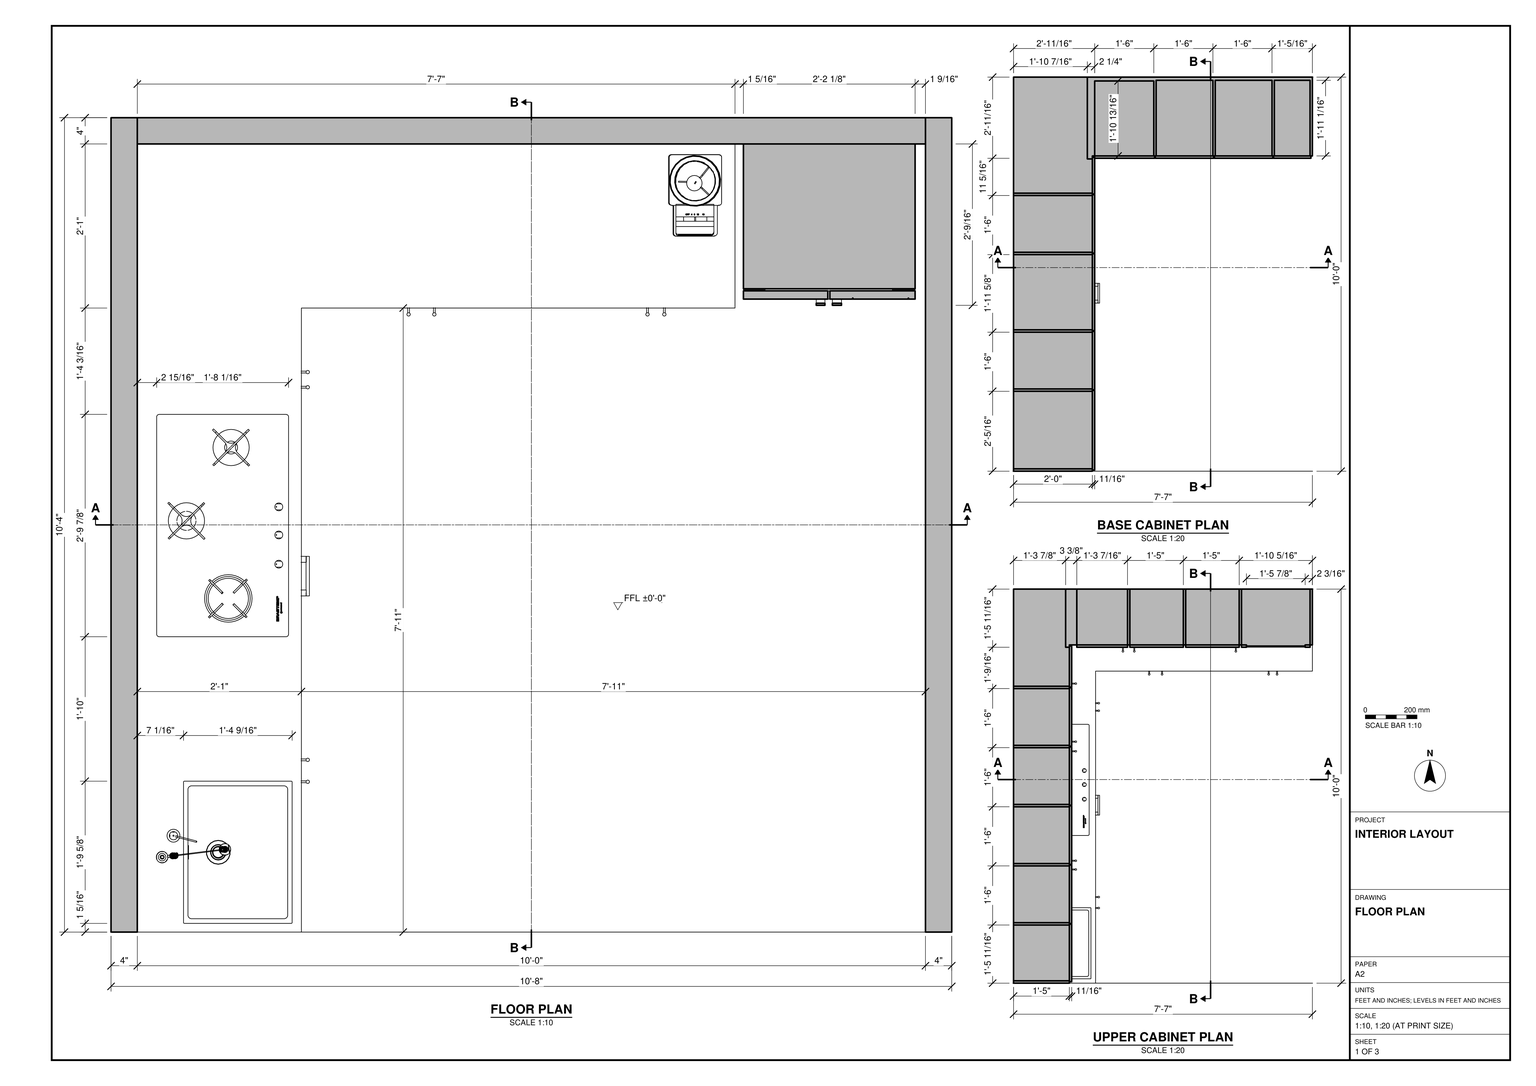
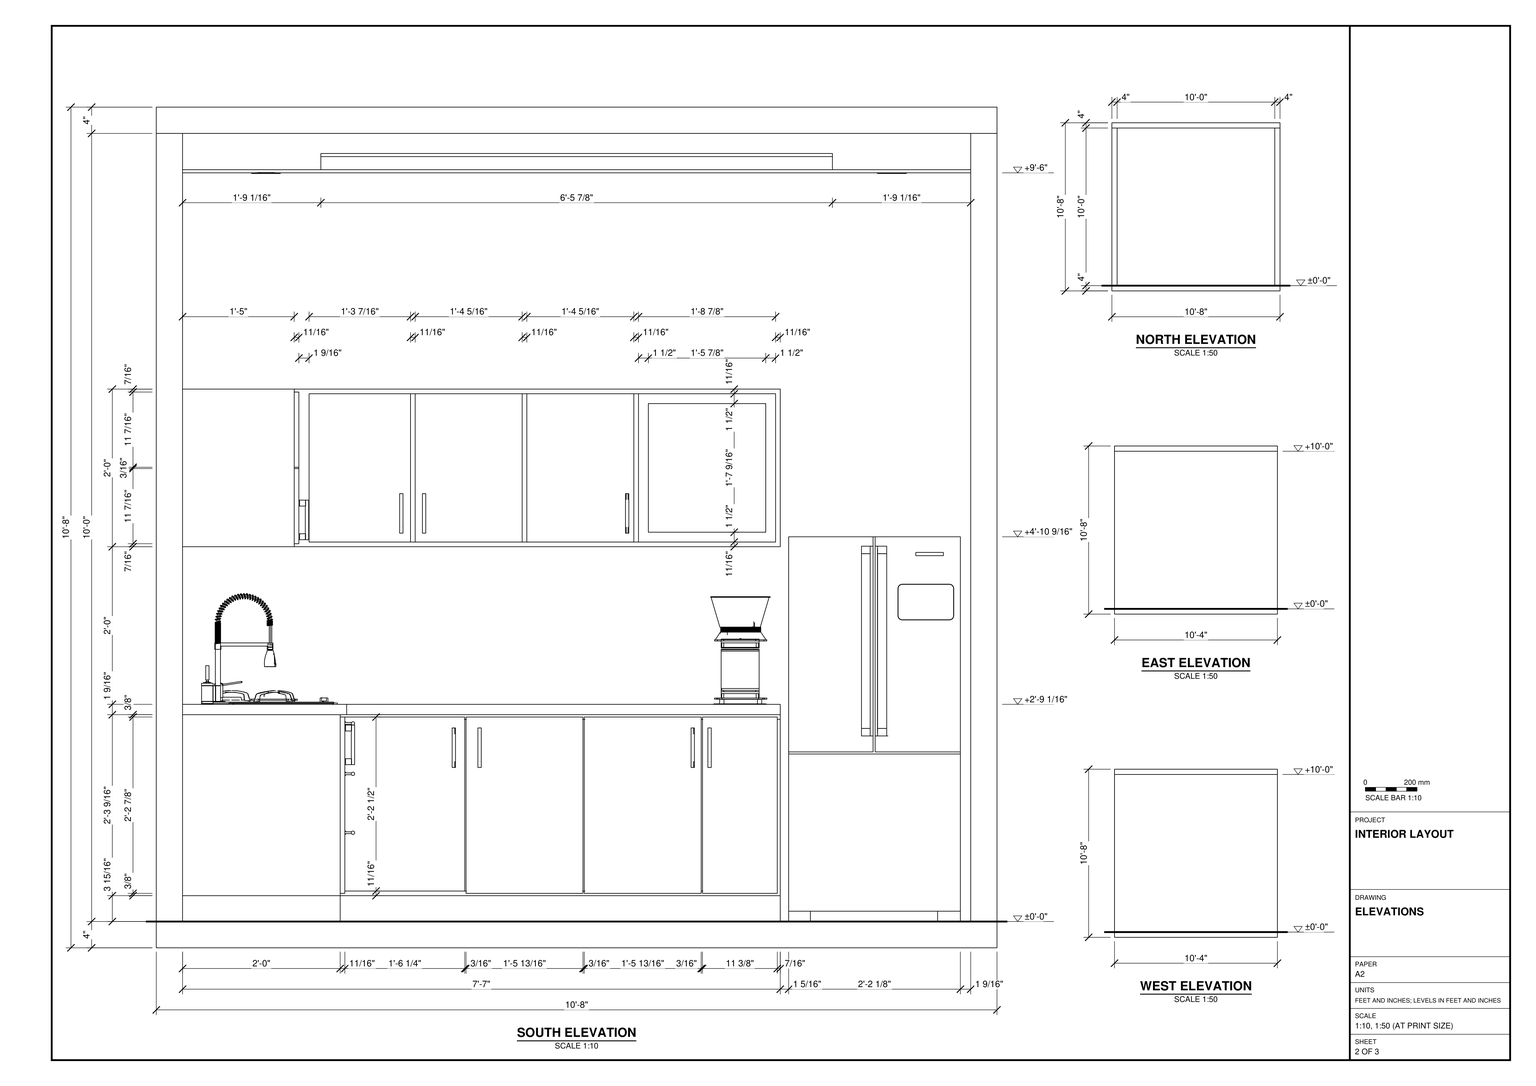
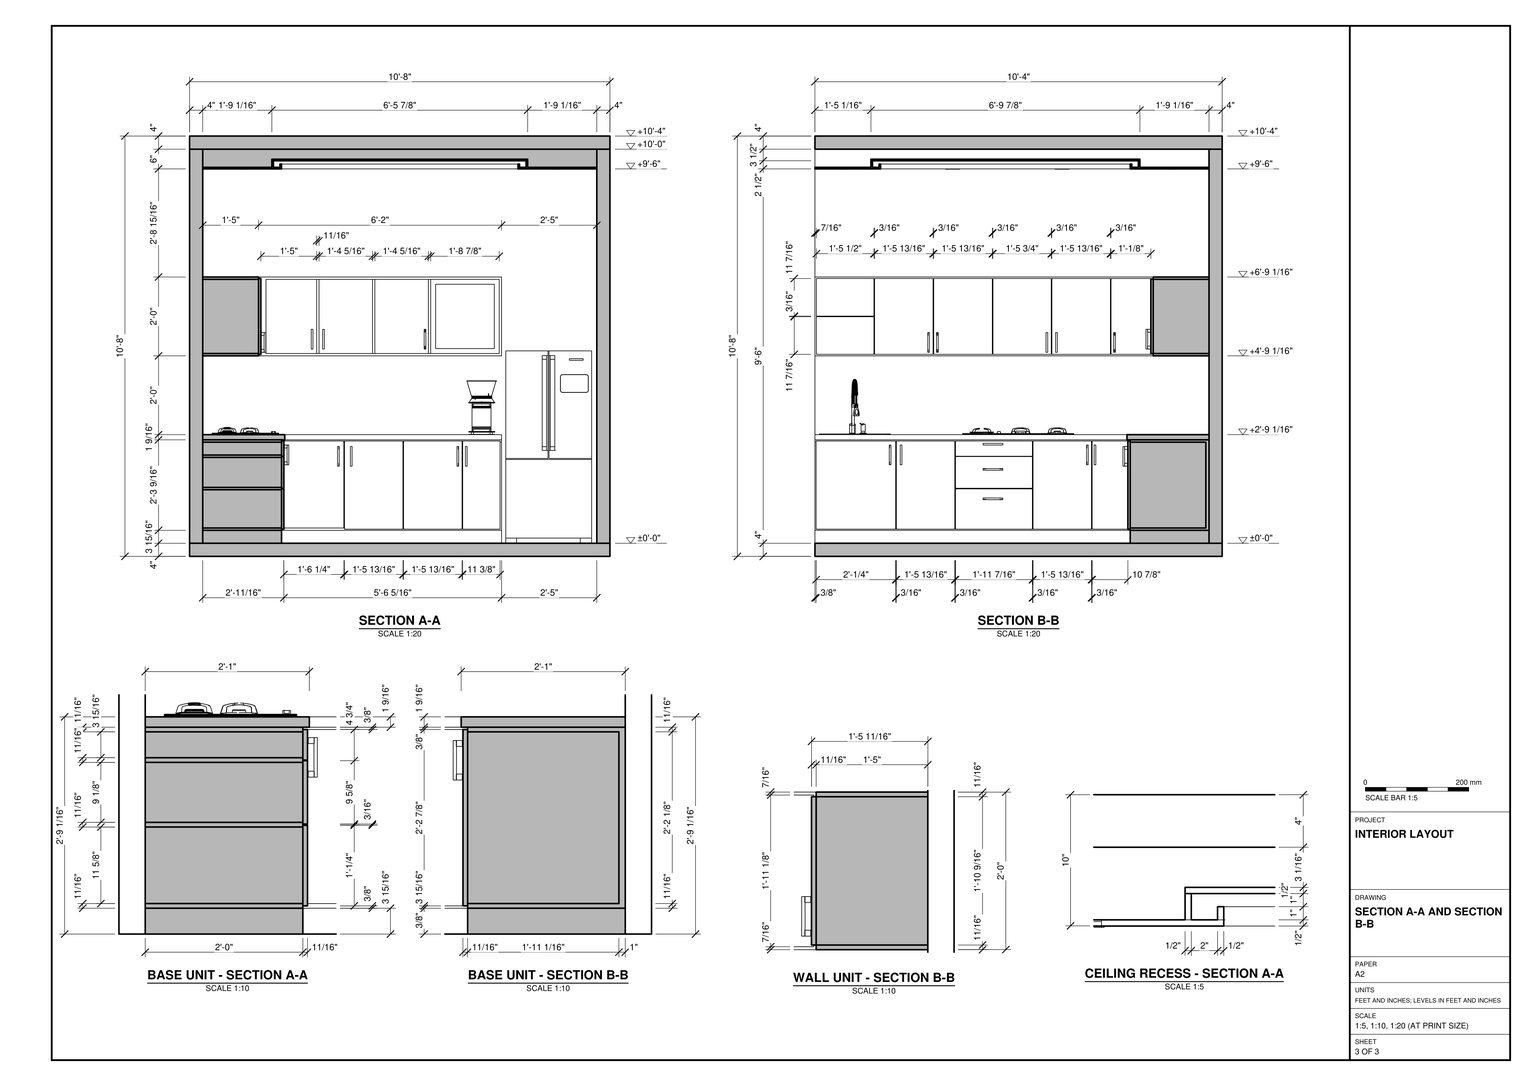
Build the kitchen in SketchUp from task_files/diagram_01.pdf. Work in feet and inches. The overall model is 10'-8" wide, 10'-4" deep and 10'-8" high, with the finished floor at ±0'-0". Model the floor slab, the 4" side and rear walls, and the overhead slab. Leave the front open as shown in plan. Use the sections to form the stepped rectangular recess in the ceiling below the overhead slab.

Fit the longer cabinet run against the left wall and turn the shorter run along the rear wall, leaving space at its right end for the refrigerator. Use the separate base and upper cabinet plans to set out the corner, cabinet depths and divisions. Model the plinths, worktop, cabinet fronts and handles to match the elevations. Place the sink and tap near the open end of the left worktop, the cooktop above the drawer bank and the small countertop appliance near the refrigerator. Decor and loose items, including appliances, may be any suitable library components.

Keep the walls, slabs, recessed ceiling and each furniture or joinery piece in separate groups or components, and use components for repeated parts. Save one SketchUp model as output_files/l_shaped_fitted_kitchen_with_recessed_ceiling.skp.

# SketchUp Ruby script. Lengths in inches.
U = 1.inch
M = Sketchup.active_model
def pt(a) = Geom::Point3d.new(a.map { |v| v * U })
def face(e, loops, mat)
  f = e.add_face(loops[0].map { |a| pt(a) })
  loops[1..].each { |l| e.add_face(l.map { |a| pt(a) }).erase! }
  f.material = f.back_material = mat if mat
  f
end
# faces: each face lists its corners as indices into pts; further lists are holes
def faces(e, pts, list, mat = nil) = list.each { |f| face(e, (f[0].is_a?(Array) ? f : [f]).map { |l| l.map { |i| pts[i] } }, mat) }
# xy, xz, yz: faces in a plane at the given z, y or x. An outline is a flat list of corners, or four numbers for a rectangle; further outlines are holes
def ring(l) = l.size == 4 ? [[l[0], l[1]], [l[2], l[1]], [l[2], l[3]], [l[0], l[3]]] : l.each_slice(2).to_a
def flat(e, list, mat, &to3) = list.each { |f| face(e, (f[0].is_a?(Array) ? f : [f]).map { |l| ring(l).map { |u, v| to3.(u, v) } }, mat) }
def xy(e, z, list, mat = nil) = flat(e, list, mat) { |x, y| [x, y, z] }
def xz(e, y, list, mat = nil) = flat(e, list, mat) { |x, z| [x, y, z] }
def yz(e, x, list, mat = nil) = flat(e, list, mat) { |y, z| [x, y, z] }
def lines(e, pts, list) = list.each { |a, b| e.add_line(pt(pts[a]), pt(pts[b])) }
# prism: a flat outline (further loops are holes) pulled along v
def prism(e, loops, v, mat = nil)
  f = face(e, loops, mat); d = Geom::Vector3d.new(v.map { |x| x * U })
  f.pushpull(f.normal.samedirection?(d) ? d.length : -d.length)
end
def box(e, o, s, mat = nil) = prism(e, [[o, [o[0] + s[0], o[1], o[2]], [o[0] + s[0], o[1] + s[1], o[2]], [o[0], o[1] + s[1], o[2]]]], [0, 0, s[2]], mat)
def at(x, y, z, deg = 0) = Geom::Transformation.translation(pt([x, y, z])) * Geom::Transformation.rotation(ORIGIN, Z_AXIS, deg.degrees)
def axes(o, x, y, z) = Geom::Transformation.new([*x, 0, *y, 0, *z, 0, *pt(o).to_a, 1])
def part(name) = M.definitions.add(name)
# library, detail: a bought-in or finely detailed component or shape, given as its bounding box
def library(name, o, s) = part(name).tap { |d| box(d.entities, o, s) }
def detail(e, o, s) = box(e.add_group.entities, o, s)
def put(e, d, t, mat = nil) = e.add_instance(d, t).tap { |i| i.material = mat if mat }
def group(e, t, mat = nil) = e.add_group.tap { |g| g.transformation = t; g.material = mat if mat }.entities
root = M.entities
M.materials.add("Marble White 100cm").color = [222, 222, 222]
M.materials.add("Tiles Simple 02 100cm").color = [183, 183, 183]
M.materials.add("base cabinate colour").color = [192, 148, 199]
M.materials.add("cabinate colour").color = [171, 171, 171]
M.materials.add("clear glass").color = [0, 0, 0]
c1 = library("geladeira side by side",[0,0,0],[32.68,30.71,73.23])
c2 = library("Kitchen sink assembly",[0,0,0],[21.65,23.57,24.55])
c3 = library("9-POIGNEE CLC2",[-3.01,-0.26,0],[6.02,0.52,1.49])
c4 = library("7-TABLE DE CUISSON CLC2",[-16.93,-10.04,0.13],[33.86,20.08,1.97])
c5 = library("Group\#15",[0,4,-0.1],[120,120,2.57])
c6 = library("Group\#38",[0,0,0],[9.87,6.84,12.32])
p = [[4,120,0],[4,0,0],[124,0,0],[124,120,0],[21,0.71,80.36],[21,0,80.36],
  [94.29,103,80.36],[95,103,80.36]]
lines(root,p,[[0,1],[2,3],[3,0],[4,5],[6,7]])
put(root,c1,axes([96.28,95.43,0],[0.8,0,0],[0,0.8,0],[0,0,0.8]))
put(root,c2,at(27.57,1.32,25.41,90))
put(root,c3,axes([28.71,22.89,26.9],[0,0,-1],[0,1,0],[1,0,0]))
put(root,c3,axes([28.71,26.22,26.9],[0,0,-1],[0,1,0],[1,0,0]))
put(root,c3,axes([28.71,82.96,26.9],[0,0,-1],[0,1,0],[1,0,0]))
put(root,c3,axes([28.71,85.27,26.9],[0,0,-1],[0,1,0],[1,0,0]))
put(root,c3,axes([28.71,54.19,30.17],[0,1,0],[0,0,1],[1,0,0]))
put(root,c3,axes([28.71,54.19,22.49],[0,1,0],[0,0,1],[1,0,0]))
put(root,c3,axes([28.71,54.19,13.52],[0,1,0],[0,0,1],[1,0,0]))
put(root,c3,axes([45.3,95.29,26.47],[0,0,-1],[1,0,0],[0,-1,0]))
put(root,c3,axes([49.22,95.29,26.47],[0,0,-1],[1,0,0],[0,-1,0]))
put(root,c3,axes([81.68,95.29,26.47],[0,0,-1],[1,0,0],[0,-1,0]))
put(root,c3,axes([84.24,95.29,26.47],[0,0,-1],[1,0,0],[0,-1,0]))
put(root,c3,axes([71.69,102.29,62.15],[0,0,-1],[1,0,0],[0,-1,0]))
put(root,c3,axes([40.77,102.29,62.15],[0,0,-1],[1,0,0],[0,-1,0]))
put(root,c3,axes([37.31,102.29,62.15],[0,0,-1],[1,0,0],[0,-1,0]))
put(root,c3,axes([21.71,34.62,61.15],[0,0,-1],[0,1,0],[1,0,0]))
put(root,c3,axes([21.71,37.28,61.15],[0,0,-1],[0,1,0],[1,0,0]))
put(root,c3,axes([21.71,70.62,61.15],[0,0,-1],[0,1,0],[1,0,0]))
put(root,c3,axes([21.71,73.54,61.15],[0,0,-1],[0,1,0],[1,0,0]))
put(root,c3,axes([21.71,91.22,61.15],[0,0,-1],[0,1,0],[1,0,0]))
put(root,c4,at(16.99,61.9,33.07,90))
g1 = group(root,at(124,-4,0))
box(g1,[0,4,0],[4,124,120])
g2 = group(root,at(4,120,0))
box(g2,[0,0,0],[120,4,120])
g3 = group(root,at(0,-4,0))
box(g3,[0,4,0],[4,124,120])
g4 = group(root,at(0,0,120))
box(g4,[0,0,0],[128,124,4])
g5 = group(root,at(0,0,-4))
xy(g5,0,[[0,0,128,124]])
xy(g5,4,[[0,0,128,124]],"Tiles Simple 02 100cm")
xz(g5,0,[[0,0,128,4]])
xz(g5,124,[[0,0,128,4]])
yz(g5,0,[[0,0,124,4]])
yz(g5,128,[[0,0,124,4]])
g6 = group(root,at(4,0,0),"Marble White 100cm")
prism(g6,[[[24,96,0],[24,0,0],[0,0,0],[0,120,0],[91,120,0],[91,96,0]]],[0,0,3.9375])
g7 = group(root,at(4,0,3.9375),"cabinate colour")
xy(g7,0,[[0,0,0,120,91,120,91,96,24,96,24,0]])
xy(g7,0.71,[[0,0.71,24,24.33],[0,25.04,24,42.33],[0,43.04,24,65.95],[0,66.66,24,83.95],[0,84.66,24,84.66,24,95.09,22.47,95.09,22.47,120,0,120],
  [24.71,96,42.71,118.83],[43.42,96,60.71,119.03],[61.42,96,78.71,119.03],[79.42,96,90.29,119.03]])
xy(g7,12.36,[[0,43.04,24,65.95]])
xy(g7,13.07,[[0,43.04,24,65.95]])
xy(g7,22.2,[[0,43.04,24,65.95]])
xy(g7,22.91,[[0,43.04,24,65.95]])
xy(g7,26.85,[[0,25.04,24,42.33],[0,43.04,24,65.95],[0,66.66,24,83.95],[0,84.66,0,120,22.47,120,22.47,95.09,24,95.09,24,84.66],[24.71,96,42.71,118.83],
  [43.42,96,60.71,119.03],[61.42,96,78.71,119.03],[79.42,96,90.29,119.03]])
xy(g7,27.56,[[[0,0,24,0,24,96,91,96,91,120,0,120],[8.17,2.03,8.01,2.1,7.96,2.125,7.84,2.24,7.8,2.28,7.73,2.4375,7.71,2.49,7.71,21.81,7.78,21.97,7.8,22.02,7.91,22.14,7.96,22.18,8.11,22.25,8.17,22.27,22.4375,22.27,22.6,22.2,22.65,22.18,22.77,22.0625,22.81,22.02,22.875,21.87,22.9,21.81,22.9,2.49,22.83,2.34,22.81,2.28,22.69,2.16,22.65,2.125,22.49,2.06,22.4375,2.03]]])
xz(g7,0,[[0,0,24,27.56]])
xz(g7,0.71,[[0,0.71,24,26.85]])
xz(g7,24.33,[[0,0.71,24,26.85]])
xz(g7,25.04,[[0,0.71,24,26.85]])
xz(g7,42.33,[[0,0.71,24,26.85]])
xz(g7,43.04,[[0,0.71,24,12.36],[0,13.07,24,22.2],[0,22.91,24,26.85]])
xz(g7,65.95,[[0,0.71,24,12.36],[0,13.07,24,22.2],[0,22.91,24,26.85]])
xz(g7,66.66,[[0,0.71,24,26.85]])
xz(g7,83.95,[[0,0.71,24,26.85]])
xz(g7,84.66,[[0,0.71,24,26.85]])
xz(g7,95.09,[[22.47,0.71,24,26.85]])
xz(g7,96,[[24,0,91,0,91,26.85,90.29,26.85,90.29,0.71,24.71,0.71,24.71,26.85,24,26.85],[42.71,0.71,43.42,26.85],[60.71,0.71,61.42,26.85],[78.71,0.71,79.42,26.85],[24,26.85,91,27.56]])
xz(g7,118.83,[[24.71,0.71,42.71,26.85]])
xz(g7,119.03,[[43.42,0.71,60.71,26.85],[61.42,0.71,78.71,26.85],[79.42,0.71,90.29,26.85]])
xz(g7,120,[[0,0,0,0.71,22.47,0.71,22.47,26.85,0,26.85,0,27.56,91,27.56,91,0]])
yz(g7,0,[[[0,0,0,27.56,120,27.56,120,26.85,84.66,26.85,84.66,0.71,120,0.71,120,0],[0.71,0.71,24.33,26.85],[66.66,0.71,83.95,26.85],[25.04,0.71,42.33,26.85],[43.04,0.71,65.95,12.36],[43.04,13.07,65.95,22.2],[43.04,22.91,65.95,26.85]]])
yz(g7,22.47,[[95.09,0.71,120,26.85]])
yz(g7,24,[[0,0,96,0,96,26.85,95.09,26.85,95.09,0.71,0.71,0.71,0.71,26.85,0,26.85],[24.33,0.71,25.04,26.85],[42.33,0.71,43.04,26.85],[65.95,0.71,66.66,26.85],[83.95,0.71,84.66,26.85],
  [43.04,12.36,65.95,13.07],[43.04,22.2,65.95,22.91],[0,26.85,96,27.56]])
yz(g7,24.71,[[96,0.71,118.83,26.85]])
yz(g7,42.71,[[96,0.71,118.83,26.85]])
yz(g7,43.42,[[96,0.71,119.03,26.85]])
yz(g7,60.71,[[96,0.71,119.03,26.85]])
yz(g7,61.42,[[96,0.71,119.03,26.85]])
yz(g7,78.71,[[96,0.71,119.03,26.85]])
yz(g7,79.42,[[96,0.71,119.03,26.85]])
yz(g7,90.29,[[96,0.71,119.03,26.85]])
yz(g7,91,[[96,0,120,27.56]])
g8 = group(root,at(4,0,31.5),"Marble White 100cm")
xy(g8,0,[[[0,0,0,120,91,120,91,96,24,96,24,0],[8.17,2.03,22.4375,2.03,22.49,2.06,22.65,2.125,22.69,2.16,22.81,2.28,22.83,2.34,22.9,2.49,22.9,21.81,22.875,21.87,22.81,22.02,22.77,22.0625,22.65,22.18,22.6,22.2,22.4375,22.27,8.17,22.27,8.11,22.25,7.96,22.18,7.91,22.14,7.8,22.02,7.78,21.97,7.71,21.81,7.71,2.49,7.73,2.4375,7.8,2.28,7.84,2.24,7.96,2.125,8.01,2.1]],[24,0,24,96,91,96,91,95.02,24.98,95.02,24.98,0]],"Marble White 100cm")
xy(g8,1.57,[[[0,0,24.98,0,24.98,95.02,91,95.02,91,120,0,120],[8.17,2.03,7.96,2.12,7.96,2.125,7.71,21.81,7.95,22.18,7.96,22.18,8.16,22.27,22.4375,22.27,22.81,22.03,22.81,22.02,22.9,21.8125,22.9,2.49,22.44,2.04,22.4375,2.03]]],"Marble White 100cm")
xz(g8,0,[[0,0,24.98,1.57]],"Marble White 100cm")
xz(g8,95.02,[[24.98,0,91,1.57]],"Marble White 100cm")
xz(g8,120,[[0,0,91,1.57]],"Marble White 100cm")
yz(g8,0,[[0,0,120,1.57]],"Marble White 100cm")
yz(g8,24.98,[[0,0,95.02,1.57]],"Marble White 100cm")
yz(g8,91,[[95.02,0,120,1.57]],"Marble White 100cm")
g9 = group(root,at(28,0.35,4.29),"base cabinate colour")
box(g9,[0,0,0],[0.71,24.23,26.85])
box(g9,[0,24.43,0],[0.71,17.8,26.85])
box(g9,[0,42.43,22.2],[0.71,23.42,4.65])
box(g9,[0,42.43,12.46],[0.71,23.42,9.65])
box(g9,[0,42.43,0],[0.71,23.42,12.26])
box(g9,[0,66.05,0],[0.71,17.8,26.85])
box(g9,[0,84.05,0],[0.71,11.14,26.85])
g10 = group(root,at(28.71,95.29,4.65),"base cabinate colour")
box(g10,[0,0,0],[18.26,0.71,26.5])
g11 = group(root,at(47.16,95.29,4.29),"base cabinate colour")
box(g11,[0,0,0],[17.8,0.71,26.85])
g12 = group(root,at(65.16,95.29,4.29),"base cabinate colour")
box(g12,[0,0,0],[17.8,0.71,26.85])
g13 = group(root,at(83.16,95.29,4.29),"base cabinate colour")
box(g13,[0,0,0],[11.39,0.71,26.85])
g14 = group(root,at(4,0,57.07),"cabinate colour")
xy(g14,0,[[0,0,0,120,91,120,91,103,17,103,17,0]])
xy(g14,0.71,[[0,0.71,17,17.71],[0,18.42,17,35.71],[0,36.42,17,53.71],[0,54.42,17,71.71],[0,72.42,17,89.71],
  [0,90.42,17,90.42,17,102.29,15.86,102.29,15.86,120,0,120],[19.26,103,34.71,120],[35.42,103,51.71,120],[52.42,103,68.71,120],[69.42,103,90.29,120]])
xy(g14,11.65,[[0,0.71,16.02,17.71],[69.42,103.98,90.29,120]])
xy(g14,12.35,[[0,0.71,16.02,17.71],[69.42,103.98,90.29,120]])
xy(g14,23.29,[[0,0.71,17,17.71],[0,18.42,17,35.71],[0,36.42,17,53.71],[0,54.42,17,71.71],[0,72.42,17,89.71],
  [0,90.42,0,120,15.86,120,15.86,102.29,17,102.29,17,90.42],[19.26,103,34.71,120],[35.42,103,51.71,120],[52.42,103,68.71,120],[69.42,103,90.29,120]])
xy(g14,24,[[0,0,17,0,17,103,91,103,91,120,0,120]])
xz(g14,0,[[0,0,17,24]])
xz(g14,0.71,[[0,0.71,17,11.65],[16.02,11.65,17,12.35],[0,12.35,17,23.29]])
xz(g14,17.71,[[0,0.71,17,11.65],[16.02,11.65,17,12.35],[0,12.35,17,23.29]])
xz(g14,18.42,[[0,0.71,17,23.29]])
xz(g14,35.71,[[0,0.71,17,23.29]])
xz(g14,36.42,[[0,0.71,17,23.29]])
xz(g14,53.71,[[0,0.71,17,23.29]])
xz(g14,54.42,[[0,0.71,17,23.29]])
xz(g14,71.71,[[0,0.71,17,23.29]])
xz(g14,72.42,[[0,0.71,17,23.29]])
xz(g14,89.71,[[0,0.71,17,23.29]])
xz(g14,90.42,[[0,0.71,17,23.29]])
xz(g14,102.29,[[15.86,0.71,17,23.29]])
xz(g14,103,[[[17,0,91,24],[19.26,0.71,90.29,23.29]],[34.71,0.71,35.42,23.29],[51.71,0.71,52.42,23.29],[68.71,0.71,69.42,23.29]])
xz(g14,103.98,[[69.42,11.65,90.29,12.35]])
xz(g14,120,[[[0,0,0,0.71,15.86,0.71,15.86,23.29,0,23.29,0,24,91,24,91,0],[52.42,0.71,68.71,23.29],[35.42,0.71,51.71,23.29],[19.26,0.71,34.71,23.29],[69.42,0.71,90.29,11.65],[69.42,12.35,90.29,23.29]]])
yz(g14,0,[[[0,0,0,24,120,24,120,23.29,90.42,23.29,90.42,0.71,120,0.71,120,0],[36.42,0.71,53.71,23.29],[54.42,0.71,71.71,23.29],[72.42,0.71,89.71,23.29],[18.42,0.71,35.71,23.29],[0.71,12.35,17.71,23.29],[0.71,0.71,17.71,11.65]]])
yz(g14,15.86,[[102.29,0.71,120,23.29]])
yz(g14,16.02,[[0.71,11.65,17.71,12.35]])
yz(g14,17,[[[0,0,103,24],[72.42,0.71,89.71,23.29],[54.42,0.71,71.71,23.29],[36.42,0.71,53.71,23.29],[18.42,0.71,35.71,23.29],[0.71,0.71,17.71,23.29],[90.42,0.71,102.29,23.29]]])
yz(g14,19.26,[[103,0.71,120,23.29]])
yz(g14,34.71,[[103,0.71,120,23.29]])
yz(g14,35.42,[[103,0.71,120,23.29]])
yz(g14,51.71,[[103,0.71,120,23.29]])
yz(g14,52.42,[[103,0.71,120,23.29]])
yz(g14,68.71,[[103,0.71,120,23.29]])
yz(g14,69.42,[[103,0.71,120,11.65],[103,11.65,103.98,12.35],[103,12.35,120,23.29]])
yz(g14,90.29,[[103,0.71,120,11.65],[103,11.65,103.98,12.35],[103,12.35,120,23.29]])
yz(g14,91,[[103,0,120,24]])
g15 = group(root,at(21,0.45,69.17),"base cabinate colour")
box(g15,[0,0,0],[0.71,17.51,11.45])
box(g15,[0,0,-11.65],[0.71,17.51,11.45])
box(g15,[0,17.71,-11.65],[0.71,17.8,23.1])
box(g15,[0,35.71,-11.65],[0.71,17.84,23.1])
box(g15,[0,53.75,-11.65],[0.71,17.75,23.1])
box(g15,[0,71.7,-11.65],[0.71,17.81,23.1])
box(g15,[0,89.71,-11.65],[0.71,12.48,23.1])
box(g15,[2.26,101.84,-11.39],[15.45,0.71,22.58])
box(g15,[18.42,101.84,-11.39],[16.29,0.71,22.58])
box(g15,[35.42,101.84,-11.39],[16.29,0.71,22.58])
xy(g15,-11.39,[[52.42,101.84,73.29,102.55]])
xy(g15,-9.89,[[53.92,101.84,71.79,102.19],[53.92,102.19,71.79,102.55]])
xy(g15,9.69,[[53.92,101.84,71.79,102.19],[53.92,102.19,71.79,102.55]])
xy(g15,11.19,[[52.42,101.84,73.29,102.55]])
xz(g15,101.84,[[[52.42,-11.39,73.29,11.19],[53.92,-9.89,71.79,9.69]]])
xz(g15,102.55,[[[52.42,-11.39,73.29,11.19],[53.92,-9.89,71.79,9.69]]])
yz(g15,52.42,[[101.84,-11.39,102.55,11.19]])
yz(g15,53.92,[[101.84,-9.89,102.19,9.69],[102.19,-9.89,102.55,9.69]])
yz(g15,71.79,[[101.84,-9.89,102.19,9.69],[102.19,-9.89,102.55,9.69]])
yz(g15,73.29,[[101.84,-11.39,102.55,11.19]])
g16 = group(g15,at(53.92,102.19,-9.89),"clear glass")
xz(g16,0,[[0,0,17.875,19.58]])
put(root,c5,at(4,-4,114))
g17 = group(root,at(25.06,17.06,116.47))
box(g17,[0,0,0],[77.89,81.89,0.47])
put(root,c6,axes([84.41,119.08,33.07],[0,-1.33,0],[1.33,0,0],[0,0,1.33]))
